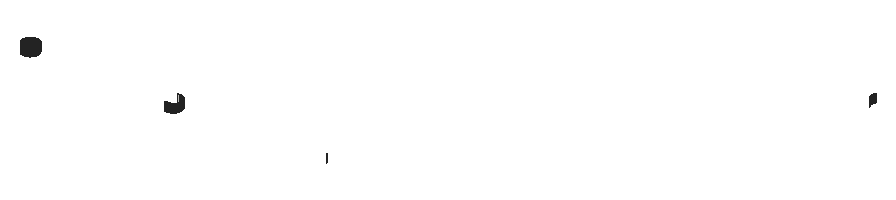
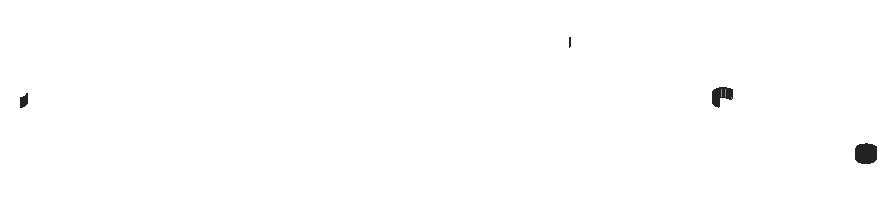
# SketchUp Ruby script. Lengths in inches.
U = 1.inch
M = Sketchup.active_model
def pt(a) = Geom::Point3d.new(a.map { |v| v * U })
def face(e, loops, mat)
  f = e.add_face(loops[0].map { |a| pt(a) })
  loops[1..].each { |l| e.add_face(l.map { |a| pt(a) }).erase! }
  f.material = f.back_material = mat if mat
  f
end
# faces: each face lists its corners as indices into pts; further lists are holes
def faces(e, pts, list, mat = nil) = list.each { |f| face(e, (f[0].is_a?(Array) ? f : [f]).map { |l| l.map { |i| pts[i] } }, mat) }
# xy, xz, yz: faces in a plane at the given z, y or x. An outline is a flat list of corners, or four numbers for a rectangle; further outlines are holes
def ring(l) = l.size == 4 ? [[l[0], l[1]], [l[2], l[1]], [l[2], l[3]], [l[0], l[3]]] : l.each_slice(2).to_a
def flat(e, list, mat, &to3) = list.each { |f| face(e, (f[0].is_a?(Array) ? f : [f]).map { |l| ring(l).map { |u, v| to3.(u, v) } }, mat) }
def xy(e, z, list, mat = nil) = flat(e, list, mat) { |x, y| [x, y, z] }
def xz(e, y, list, mat = nil) = flat(e, list, mat) { |x, z| [x, y, z] }
def yz(e, x, list, mat = nil) = flat(e, list, mat) { |y, z| [x, y, z] }
def lines(e, pts, list) = list.each { |a, b| e.add_line(pt(pts[a]), pt(pts[b])) }
# prism: a flat outline (further loops are holes) pulled along v
def prism(e, loops, v, mat = nil)
  f = face(e, loops, mat); d = Geom::Vector3d.new(v.map { |x| x * U })
  f.pushpull(f.normal.samedirection?(d) ? d.length : -d.length)
end
def box(e, o, s, mat = nil) = prism(e, [[o, [o[0] + s[0], o[1], o[2]], [o[0] + s[0], o[1] + s[1], o[2]], [o[0], o[1] + s[1], o[2]]]], [0, 0, s[2]], mat)
def at(x, y, z, deg = 0) = Geom::Transformation.translation(pt([x, y, z])) * Geom::Transformation.rotation(ORIGIN, Z_AXIS, deg.degrees)
def axes(o, x, y, z) = Geom::Transformation.new([*x, 0, *y, 0, *z, 0, *pt(o).to_a, 1])
def part(name) = M.definitions.add(name)
# library, detail: a bought-in or finely detailed component or shape, given as its bounding box
def library(name, o, s) = part(name).tap { |d| box(d.entities, o, s) }
def detail(e, o, s) = box(e.add_group.entities, o, s)
def put(e, d, t, mat = nil) = e.add_instance(d, t).tap { |i| i.material = mat if mat }
def group(e, t, mat = nil) = e.add_group.tap { |g| g.transformation = t; g.material = mat if mat }.entities
root = M.entities
xz(root,185,[[49.875,231,49.95,234],[49.95,231,50.03,234],[50.03,231,50.11,234],[104.68,231,104.75,234],[104.75,231,104.83,234],
  [104.83,231,104.91,234]])
xz(root,185.01,[[49.72,231,49.8,234],[50.19,231,50.27,234],[104.52,231,104.6,234],[104.99,231,105.07,234]])
xz(root,190.99,[[49.73,231,49.81,234],[50.2,231,50.28,234],[104.53,231,104.61,234],[105,231,105.08,234]])
xz(root,191,[[49.89,231,49.97,234],[49.97,231,50.05,234],[50.05,231,50.125,234],[104.6875,231,104.77,234],[104.77,231,104.85,234],
  [104.85,231,104.92,234]])
yz(root,47,[[187.89,231,187.97,234],[187.97,231,188.05,234],[188.05,231,188.125,234]])
yz(root,47.01,[[187.73,231,187.81,234],[188.2,231,188.28,234]])
yz(root,52.99,[[187.72,231,187.8,234],[188.19,231,188.27,234]])
yz(root,53,[[187.875,231,187.95,234],[187.95,231,188.03,234],[188.03,231,188.11,234]])
yz(root,107.79,[[187.72,231,187.8,234],[188.19,231,188.27,234]])
yz(root,107.8,[[187.875,231,187.95,234],[187.95,231,188.03,234],[188.03,231,188.11,234]])
yz(root,266.2,[[319.89,231,319.97,234],[319.97,231,320.05,234],[320.05,231,320.125,234]])
yz(root,266.21,[[319.73,231,319.81,234],[320.2,231,320.28,234]])
p = [[49.49,185.04,231],[49.41,185.06,231],[49.41,185.06,234],[49.49,185.04,234],[49.5625,185.03,231],[49.5625,185.03,234],
  [49.64,185.02,231],[49.64,185.02,234],[49.72,185.01,231],[49.72,185.01,234],[49.875,185,231],[49.8,185.01,231],
  [49.8,185.01,234],[49.875,185,234],[50.19,185.01,231],[50.11,185,231],[50.11,185,234],[50.19,185.01,234],
  [50.35,185.02,231],[50.27,185.01,231],[50.27,185.01,234],[50.35,185.02,234],[50.42,185.03,231],[50.42,185.03,234],
  [50.5,185.04,231],[50.5,185.04,234],[50.58,185.06,231],[50.58,185.06,234],[104.29,185.04,231],[104.21,185.06,231],
  [104.21,185.06,234],[104.29,185.04,234],[104.36,185.03,231],[104.36,185.03,234],[104.44,185.02,231],[104.44,185.02,234],
  [104.52,185.01,231],[104.52,185.01,234],[104.68,185,231],[104.6,185.01,231],[104.6,185.01,234],[104.68,185,234],
  [104.99,185.01,231],[104.91,185,231],[104.91,185,234],[104.99,185.01,234],[105.15,185.02,231],[105.07,185.01,231],
  [105.07,185.01,234],[105.15,185.02,234],[105.22,185.03,231],[105.22,185.03,234],[105.3,185.04,231],[105.3,185.04,234],
  [105.38,185.06,231],[105.38,185.06,234],[49.1,185.14,231],[49.03,185.16,231],[49.03,185.16,234],[49.1,185.14,234],
  [49.18,185.11,231],[49.18,185.11,234],[49.26,185.09,231],[49.26,185.09,234],[49.33,185.08,231],[49.33,185.08,234],
  [50.66,185.07,231],[50.66,185.07,234],[50.73,185.09,231],[50.73,185.09,234],[50.81,185.11,231],[50.81,185.11,234],
  [50.88,185.13,231],[50.88,185.13,234],[50.96,185.16,231],[50.96,185.16,234],[103.98,185.11,231],[103.9,185.14,231],
  [103.9,185.14,234],[103.98,185.11,234],[104.06,185.09,231],[104.06,185.09,234],[104.13,185.08,231],[104.13,185.08,234],
  [105.46,185.07,231],[105.46,185.07,234],[105.53,185.09,231],[105.53,185.09,234],[105.61,185.11,231],[105.61,185.11,234],
  [105.68,185.13,231],[105.68,185.13,234],[105.76,185.16,231],[105.76,185.16,234],[48.81,185.25,231],[48.74,185.28,231],
  [48.74,185.28,234],[48.81,185.25,234],[48.88,185.22,231],[48.88,185.22,234],[48.96,185.1875,231],[48.96,185.1875,234],
  [51.03,185.18,231],[51.03,185.18,234],[51.11,185.21,231],[51.11,185.21,234],[51.18,185.24,231],[51.18,185.24,234],
  [51.25,185.27,231],[51.25,185.27,234],[105.83,185.18,231],[105.83,185.18,234],[105.91,185.21,231],[105.91,185.21,234],
  [105.98,185.24,231],[105.98,185.24,234],[106.05,185.27,231],[106.05,185.27,234],[48.6,185.35,231],[48.53,185.39,231],
  [48.53,185.39,234],[48.6,185.35,234],[48.67,185.3125,231],[48.67,185.3125,234],[51.32,185.31,231],[51.32,185.31,234],
  [51.39,185.34,231],[51.39,185.34,234],[51.46,185.38,231],[51.46,185.38,234],[106.12,185.31,231],[106.12,185.31,234],
  [106.19,185.34,231],[106.19,185.34,234],[106.26,185.38,231],[106.26,185.38,234],[48.46,185.42,231],[48.39,185.47,231],
  [48.39,185.47,234],[48.46,185.42,234],[51.53,185.42,231],[51.53,185.42,234],[51.6,185.46,231],[51.6,185.46,234],
  [106.33,185.42,231],[106.33,185.42,234],[106.4,185.46,231],[106.4,185.46,234],[48.33,185.51,231],[48.26,185.55,231],
  [48.26,185.55,234],[48.33,185.51,234],[51.66,185.5,231],[51.66,185.5,234],[51.73,185.55,231],[51.73,185.55,234],
  [51.79,185.59,231],[51.79,185.59,234],[106.46,185.5,231],[106.46,185.5,234],[106.53,185.55,231],[106.53,185.55,234],
  [106.59,185.59,231],[106.59,185.59,234],[48.14,185.65,231],[48.08,185.7,231],[48.08,185.7,234],[48.14,185.65,234],
  [48.2,185.6,231],[48.2,185.6,234],[51.85,185.64,231],[51.85,185.64,234],[51.91,185.69,231],[51.91,185.69,234],
  [106.65,185.64,231],[106.65,185.64,234],[106.71,185.69,231],[106.71,185.69,234],[48.02,185.75,231],[47.96,185.8,231],
  [47.96,185.8,234],[48.02,185.75,234],[51.97,185.74,231],[51.97,185.74,234],[52.03,185.79,231],[52.03,185.79,234],
  [106.77,185.74,231],[106.77,185.74,234],[106.83,185.79,231],[106.83,185.79,234],[47.9,185.86,231],[47.9,185.86,234],
  [52.09,185.85,231],[52.09,185.85,234],[52.14,185.9,231],[52.14,185.9,234],[106.89,185.85,231],[106.89,185.85,234],
  [106.94,185.9,231],[106.94,185.9,234],[47.85,185.91,231],[47.79,185.97,231],[47.79,185.97,234],[47.85,185.91,234],
  [52.2,185.96,231],[52.2,185.96,234],[107,185.96,231],[107,185.96,234],[47.74,186.03,231],[47.69,186.09,231],
  [47.69,186.09,234],[47.74,186.03,234],[52.25,186.02,231],[52.25,186.02,234],[52.3,186.08,231],[52.3,186.08,234],
  [107.05,186.02,231],[107.05,186.02,234],[107.1,186.08,231],[107.1,186.08,234],[47.64,186.15,231],[47.59,186.21,231],
  [47.59,186.21,234],[47.64,186.15,234],[52.35,186.14,231],[52.35,186.14,234],[52.4,186.2,231],[52.4,186.2,234],
  [107.15,186.14,231],[107.15,186.14,234],[107.2,186.2,231],[107.2,186.2,234],[47.55,186.27,231],[47.55,186.27,234],
  [52.45,186.26,231],[52.45,186.26,234],[107.25,186.26,231],[107.25,186.26,234],[47.5,186.34,231],[47.46,186.4,231],
  [47.46,186.4,234],[47.5,186.34,234],[52.49,186.33,231],[52.49,186.33,234],[52.53,186.39,231],[52.53,186.39,234],
  [107.29,186.33,231],[107.29,186.33,234],[107.33,186.39,231],[107.33,186.39,234],[47.42,186.47,231],[47.42,186.47,234],
  [52.58,186.46,231],[52.58,186.46,234],[107.375,186.46,231],[107.375,186.46,234],[47.38,186.54,231],[47.34,186.61,231],
  [47.34,186.61,234],[47.38,186.54,234],[52.61,186.53,231],[52.61,186.53,234],[52.65,186.6,231],[52.65,186.6,234],
  [107.41,186.53,231],[107.41,186.53,234],[107.45,186.6,231],[107.45,186.6,234],[47.31,186.68,231],[47.31,186.68,234],
  [52.6875,186.67,231],[52.6875,186.67,234],[107.49,186.67,231],[107.49,186.67,234],[47.27,186.75,231],[47.24,186.82,231],
  [47.24,186.82,234],[47.27,186.75,234],[52.72,186.74,231],[52.72,186.74,234],[52.75,186.81,231],[52.75,186.81,234],
  [107.52,186.74,231],[107.52,186.74,234],[107.55,186.81,231],[107.55,186.81,234],[47.21,186.89,231],[47.21,186.89,234],
  [52.78,186.88,231],[52.78,186.88,234],[107.58,186.88,231],[107.58,186.88,234],[47.18,186.97,231],[47.18,186.97,234],
  [52.8125,186.96,231],[52.8125,186.96,234],[107.61,186.96,231],[107.61,186.96,234],[47.16,187.04,231],[47.13,187.12,231],
  [47.13,187.12,234],[47.16,187.04,234],[52.84,187.03,231],[52.84,187.03,234],[52.86,187.1,231],[52.86,187.1,234],
  [107.64,187.03,231],[107.64,187.03,234],[107.66,187.1,231],[107.66,187.1,234],[47.11,187.19,231],[47.11,187.19,234],
  [52.89,187.18,231],[52.89,187.18,234],[107.6875,187.18,231],[107.6875,187.18,234],[47.09,187.27,231],[47.09,187.27,234],
  [52.91,187.26,231],[52.91,187.26,234],[107.71,187.26,231],[107.71,187.26,234],[47.07,187.34,231],[47.06,187.42,231],
  [47.06,187.42,234],[47.07,187.34,234],[52.92,187.33,231],[52.92,187.33,234],[52.94,187.41,231],[52.94,187.41,234],
  [107.72,187.33,231],[107.72,187.33,234],[107.74,187.41,231],[107.74,187.41,234],[47.04,187.5,231],[47.04,187.5,234],
  [52.96,187.49,231],[52.96,187.49,234],[107.76,187.49,231],[107.76,187.49,234],[47.03,187.58,231],[47.03,187.58,234],
  [52.97,187.5625,231],[52.97,187.5625,234],[107.77,187.5625,231],[107.77,187.5625,234],[47.02,187.65,231],[47.02,187.65,234],
  [52.98,187.64,231],[52.98,187.64,234],[52.99,187.72,231],[52.99,187.72,234],[107.78,187.64,231],[107.78,187.64,234],
  [107.79,187.72,231],[107.79,187.72,234],[47.01,187.73,231],[47.01,187.73,234],[47.01,187.81,231],[47,187.89,231],
  [47,187.89,234],[47.01,187.81,234],[53,187.875,231],[52.99,187.8,231],[52.99,187.8,234],[53,187.875,234],
  [107.8,187.875,231],[107.79,187.8,231],[107.79,187.8,234],[107.8,187.875,234],[47,188.125,231],[47.01,188.2,231],
  [47.01,188.2,234],[47,188.125,234],[52.99,188.19,231],[53,188.11,231],[53,188.11,234],[52.99,188.19,234],
  [107.79,188.19,231],[107.8,188.11,231],[107.8,188.11,234],[107.79,188.19,234],[47.01,188.28,231],[47.02,188.36,231],
  [47.02,188.36,234],[47.01,188.28,234],[52.97,188.42,231],[52.98,188.35,231],[52.98,188.35,234],[52.97,188.42,234],
  [52.99,188.27,231],[52.99,188.27,234],[107.77,188.42,231],[107.78,188.35,231],[107.78,188.35,234],[107.77,188.42,234],
  [107.79,188.27,231],[107.79,188.27,234],[47.03,188.4375,231],[47.03,188.4375,234],[47.04,188.51,231],[47.04,188.51,234],
  [52.96,188.5,231],[52.96,188.5,234],[107.76,188.5,231],[107.76,188.5,234],[47.06,188.59,231],[47.06,188.59,234],
  [52.94,188.58,231],[52.94,188.58,234],[107.74,188.58,231],[107.74,188.58,234],[47.08,188.67,231],[47.08,188.67,234],
  [52.93,188.66,231],[52.93,188.66,234],[107.73,188.66,231],[107.73,188.66,234],[47.09,188.74,231],[47.09,188.74,234],
  [47.11,188.82,231],[47.11,188.82,234],[52.89,188.81,231],[52.91,188.73,231],[52.91,188.73,234],[52.89,188.81,234],
  [107.6875,188.81,231],[107.71,188.73,231],[107.71,188.73,234],[107.6875,188.81,234],[47.14,188.9,231],[47.14,188.9,234],
  [52.87,188.88,231],[52.87,188.88,234],[107.67,188.88,231],[107.67,188.88,234],[47.16,188.97,231],[47.16,188.97,234],
  [52.84,188.96,231],[52.84,188.96,234],[107.64,188.96,231],[107.64,188.96,234],[47.1875,189.04,231],[47.1875,189.04,234],
  [47.22,189.12,231],[47.22,189.12,234],[52.79,189.11,231],[52.82,189.03,231],[52.82,189.03,234],[52.79,189.11,234],
  [107.59,189.11,231],[107.62,189.03,231],[107.62,189.03,234],[107.59,189.11,234],[47.25,189.19,231],[47.25,189.19,234],
  [52.76,189.18,231],[52.76,189.18,234],[107.56,189.18,231],[107.56,189.18,234],[47.28,189.26,231],[47.28,189.26,234],
  [52.73,189.25,231],[52.73,189.25,234],[107.53,189.25,231],[107.53,189.25,234],[47.3125,189.33,231],[47.3125,189.33,234],
  [47.35,189.4,231],[47.35,189.4,234],[52.66,189.39,231],[52.69,189.32,231],[52.69,189.32,234],[52.66,189.39,234],
  [107.46,189.39,231],[107.49,189.32,231],[107.49,189.32,234],[107.46,189.39,234],[47.39,189.47,231],[47.39,189.47,234],
  [52.62,189.46,231],[52.62,189.46,234],[107.42,189.46,231],[107.42,189.46,234],[47.42,189.54,231],[47.42,189.54,234],
  [47.47,189.61,231],[47.47,189.61,234],[52.54,189.6,231],[52.58,189.53,231],[52.58,189.53,234],[52.54,189.6,234],
  [107.34,189.6,231],[107.38,189.53,231],[107.38,189.53,234],[107.34,189.6,234],[47.51,189.67,231],[47.51,189.67,234],
  [52.5,189.66,231],[52.5,189.66,234],[107.3,189.66,231],[107.3,189.66,234],[47.55,189.74,231],[47.55,189.74,234],
  [47.6,189.8,231],[47.6,189.8,234],[52.41,189.79,231],[52.45,189.73,231],[52.45,189.73,234],[52.41,189.79,234],
  [107.21,189.79,231],[107.25,189.73,231],[107.25,189.73,234],[107.21,189.79,234],[47.65,189.86,231],[47.65,189.86,234],
  [52.36,189.85,231],[52.36,189.85,234],[107.16,189.85,231],[107.16,189.85,234],[47.7,189.92,231],[47.7,189.92,234],
  [47.75,189.98,231],[47.75,189.98,234],[52.26,189.97,231],[52.31,189.91,231],[52.31,189.91,234],[52.26,189.97,234],
  [107.06,189.97,231],[107.11,189.91,231],[107.11,189.91,234],[107.06,189.97,234],[47.8,190.04,231],[47.8,190.04,234],
  [47.86,190.1,231],[47.86,190.1,234],[52.15,190.09,231],[52.21,190.03,231],[52.21,190.03,234],[52.15,190.09,234],
  [106.95,190.09,231],[107.01,190.03,231],[107.01,190.03,234],[106.95,190.09,234],[47.91,190.15,231],[47.91,190.15,234],
  [52.04,190.2,231],[52.1,190.14,231],[52.1,190.14,234],[52.04,190.2,234],[106.84,190.2,231],[106.9,190.14,231],
  [106.9,190.14,234],[106.84,190.2,234],[47.97,190.21,231],[47.97,190.21,234],[48.03,190.26,231],[48.03,190.26,234],
  [51.98,190.25,231],[51.98,190.25,234],[106.78,190.25,231],[106.78,190.25,234],[48.09,190.31,231],[48.09,190.31,234],
  [48.15,190.36,231],[48.15,190.36,234],[51.86,190.35,231],[51.92,190.3,231],[51.92,190.3,234],[51.86,190.35,234],
  [106.66,190.35,231],[106.72,190.3,231],[106.72,190.3,234],[106.66,190.35,234],[161.46,190.35,231],[161.52,190.3,231],
  [161.52,190.3,234],[161.46,190.35,234],[161.58,190.25,231],[161.58,190.25,234],[48.21,190.41,231],[48.21,190.41,234],
  [48.27,190.45,231],[48.27,190.45,234],[51.67,190.49,231],[51.74,190.45,231],[51.74,190.45,234],[51.67,190.49,234],
  [51.8,190.4,231],[51.8,190.4,234],[106.47,190.49,231],[106.54,190.45,231],[106.54,190.45,234],[106.47,190.49,234],
  [106.6,190.4,231],[106.6,190.4,234],[161.4,190.4,231],[161.4,190.4,234],[48.34,190.5,231],[48.34,190.5,234],
  [48.4,190.54,231],[48.4,190.54,234],[48.47,190.58,231],[48.47,190.58,234],[51.54,190.58,231],[51.61,190.53,231],
  [51.61,190.53,234],[51.54,190.58,234],[106.34,190.58,231],[106.41,190.53,231],[106.41,190.53,234],[106.34,190.58,234],
  [48.54,190.62,231],[48.54,190.62,234],[48.61,190.66,231],[48.61,190.66,234],[51.4,190.65,231],[51.47,190.61,231],
  [51.47,190.61,234],[51.4,190.65,234],[106.2,190.65,231],[106.27,190.61,231],[106.27,190.61,234],[106.2,190.65,234],
  [48.68,190.69,231],[48.68,190.69,234],[48.75,190.73,231],[48.75,190.73,234],[48.82,190.76,231],[48.82,190.76,234],
  [51.19,190.75,231],[51.26,190.72,231],[51.26,190.72,234],[51.19,190.75,234],[51.33,190.6875,231],[51.33,190.6875,234],
  [105.99,190.75,231],[106.0625,190.72,231],[106.0625,190.72,234],[105.99,190.75,234],[106.13,190.6875,231],[106.13,190.6875,234],
  [48.89,190.79,231],[48.89,190.79,234],[48.97,190.82,231],[48.97,190.82,234],[49.04,190.84,231],[49.04,190.84,234],
  [49.12,190.87,231],[49.12,190.87,234],[50.9,190.86,231],[50.97,190.84,231],[50.97,190.84,234],[50.9,190.86,234],
  [51.04,190.8125,231],[51.04,190.8125,234],[51.12,190.78,231],[51.12,190.78,234],[105.7,190.86,231],[105.77,190.84,231],
  [105.77,190.84,234],[105.7,190.86,234],[105.84,190.8125,231],[105.84,190.8125,234],[105.92,190.78,231],[105.92,190.78,234],
  [49.19,190.89,231],[49.19,190.89,234],[49.27,190.91,231],[49.27,190.91,234],[49.34,190.93,231],[49.34,190.93,234],
  [49.42,190.94,231],[49.42,190.94,234],[49.5,190.96,231],[49.5,190.96,234],[50.51,190.96,231],[50.59,190.94,231],
  [50.59,190.94,234],[50.51,190.96,234],[50.67,190.92,231],[50.67,190.92,234],[50.74,190.91,231],[50.74,190.91,234],
  [50.82,190.89,231],[50.82,190.89,234],[103.92,190.87,231],[103.99,190.89,231],[103.99,190.89,234],[103.92,190.87,234],
  [104.07,190.91,231],[104.07,190.91,234],[104.14,190.93,231],[104.14,190.93,234],[104.22,190.94,231],[104.22,190.94,234],
  [104.3,190.96,231],[104.3,190.96,234],[105.3125,190.96,231],[105.39,190.94,231],[105.39,190.94,234],[105.3125,190.96,234],
  [105.47,190.92,231],[105.47,190.92,234],[105.54,190.91,231],[105.54,190.91,234],[105.62,190.89,231],[105.62,190.89,234],
  [49.58,190.97,231],[49.58,190.97,234],[49.65,190.98,231],[49.65,190.98,234],[49.73,190.99,231],[49.73,190.99,234],
  [49.81,190.99,231],[49.89,191,231],[49.89,191,234],[49.81,190.99,234],[50.125,191,231],[50.2,190.99,231],
  [50.2,190.99,234],[50.125,191,234],[50.28,190.99,231],[50.36,190.98,231],[50.36,190.98,234],[50.28,190.99,234],
  [50.4375,190.97,231],[50.4375,190.97,234],[104.375,190.97,231],[104.375,190.97,234],[104.45,190.98,231],[104.45,190.98,234],
  [104.53,190.99,231],[104.53,190.99,234],[104.61,190.99,231],[104.6875,191,231],[104.6875,191,234],[104.61,190.99,234],
  [104.92,191,231],[105,190.99,231],[105,190.99,234],[104.92,191,234],[105.08,190.99,231],[105.16,190.98,231],
  [105.16,190.98,234],[105.08,190.99,234],[105.24,190.97,231],[105.24,190.97,234],[266.66,318.4,231],[266.62,318.47,231],
  [266.62,318.47,234],[266.66,318.4,234],[266.58,318.54,231],[266.54,318.61,231],[266.54,318.61,234],[266.58,318.54,234],
  [266.51,318.68,231],[266.51,318.68,234],[266.47,318.75,231],[266.44,318.82,231],[266.44,318.82,234],[266.47,318.75,234],
  [266.41,318.89,231],[266.41,318.89,234],[266.38,318.97,231],[266.38,318.97,234],[266.36,319.04,231],[266.33,319.12,231],
  [266.33,319.12,234],[266.36,319.04,234],[266.3125,319.19,231],[266.3125,319.19,234],[266.29,319.27,231],[266.29,319.27,234],
  [266.27,319.34,231],[266.26,319.42,231],[266.26,319.42,234],[266.27,319.34,234],[266.24,319.5,231],[266.24,319.5,234],
  [266.23,319.58,231],[266.23,319.58,234],[266.22,319.65,231],[266.22,319.65,234],[266.21,319.73,231],[266.21,319.73,234],
  [266.21,319.81,231],[266.2,319.89,231],[266.2,319.89,234],[266.21,319.81,234],[266.2,320.125,231],[266.21,320.2,231],
  [266.21,320.2,234],[266.2,320.125,234],[266.21,320.28,231],[266.22,320.36,231],[266.22,320.36,234],[266.21,320.28,234],
  [266.23,320.4375,231],[266.23,320.4375,234],[266.24,320.51,231],[266.24,320.51,234],[266.26,320.59,231],[266.26,320.59,234],
  [266.28,320.67,231],[266.28,320.67,234],[266.29,320.74,231],[266.29,320.74,234],[266.3125,320.82,231],[266.3125,320.82,234],
  [266.34,320.9,231],[266.34,320.9,234],[266.36,320.97,231],[266.36,320.97,234],[266.39,321.04,231],[266.39,321.04,234],
  [266.42,321.12,231],[266.42,321.12,234],[266.45,321.19,231],[266.45,321.19,234],[266.48,321.26,231],[266.48,321.26,234],
  [266.51,321.33,231],[266.51,321.33,234],[266.55,321.4,231],[266.55,321.4,234],[266.59,321.47,231],[266.59,321.47,234],
  [266.625,321.54,231],[266.625,321.54,234],[266.67,321.61,231],[266.67,321.61,234]]
faces(root,p,[[0,1,2,3],[4,0,3,5],[6,4,5,7],[8,6,7,9],[10,11,12,13],[14,15,16,17],[18,19,20,21],[22,18,21,23],
  [24,22,23,25],[26,24,25,27],[28,29,30,31],[32,28,31,33],[34,32,33,35],[36,34,35,37],[38,39,40,41],[42,43,44,45],
  [46,47,48,49],[50,46,49,51],[52,50,51,53],[54,52,53,55],[56,57,58,59],[60,56,59,61],[62,60,61,63],[64,62,63,65],
  [1,64,65,2],[66,26,27,67],[68,66,67,69],[70,68,69,71],[72,70,71,73],[74,72,73,75],[76,77,78,79],[80,76,79,81],
  [82,80,81,83],[29,82,83,30],[84,54,55,85],[86,84,85,87],[88,86,87,89],[90,88,89,91],[92,90,91,93],[94,95,96,97],
  [98,94,97,99],[100,98,99,101],[57,100,101,58],[102,74,75,103],[104,102,103,105],[106,104,105,107],[108,106,107,109],[110,92,93,111],
  [112,110,111,113],[114,112,113,115],[116,114,115,117],[118,119,120,121],[122,118,121,123],[95,122,123,96],[124,108,109,125],[126,124,125,127],
  [128,126,127,129],[130,116,117,131],[132,130,131,133],[134,132,133,135],[136,137,138,139],[119,136,139,120],[140,128,129,141],[142,140,141,143],
  [144,134,135,145],[146,144,145,147],[148,149,150,151],[137,148,151,138],[152,142,143,153],[154,152,153,155],[156,154,155,157],[158,146,147,159],
  [160,158,159,161],[162,160,161,163],[164,165,166,167],[168,164,167,169],[149,168,169,150],[170,156,157,171],[172,170,171,173],[174,162,163,175],
  [176,174,175,177],[178,179,180,181],[165,178,181,166],[182,172,173,183],[184,182,183,185],[186,176,177,187],[188,186,187,189],[179,190,191,180],
  [192,184,185,193],[194,192,193,195],[196,188,189,197],[198,196,197,199],[200,201,202,203],[190,200,203,191],[204,194,195,205],[206,198,199,207],
  [208,209,210,211],[201,208,211,202],[212,204,205,213],[214,212,213,215],[216,206,207,217],[218,216,217,219],[220,221,222,223],[209,220,223,210],
  [224,214,215,225],[226,224,225,227],[228,218,219,229],[230,228,229,231],[221,232,233,222],[234,226,227,235],[236,230,231,237],[238,239,240,241],
  [232,238,241,233],[242,234,235,243],[244,242,243,245],[246,236,237,247],[248,246,247,249],[239,250,251,240],[252,244,245,253],[254,248,249,255],
  [256,257,258,259],[250,256,259,251],[260,252,253,261],[262,260,261,263],[264,254,255,265],[266,264,265,267],[257,268,269,258],[270,262,263,271],
  [272,266,267,273],[274,275,276,277],[268,274,277,269],[278,270,271,279],[280,278,279,281],[282,272,273,283],[284,282,283,285],[275,286,287,276],
  [288,280,281,289],[290,284,285,291],[286,292,293,287],[294,288,289,295],[296,290,291,297],[298,299,300,301],[292,298,301,293],[302,294,295,303],
  [304,302,303,305],[306,296,297,307],[308,306,307,309],[299,310,311,300],[312,304,305,313],[314,308,309,315],[310,316,317,311],[318,312,313,319],
  [320,314,315,321],[322,323,324,325],[316,322,325,317],[326,318,319,327],[328,326,327,329],[330,320,321,331],[332,330,331,333],[323,334,335,324],
  [336,328,329,337],[338,332,333,339],[334,340,341,335],[342,336,337,343],[344,338,339,345],[340,346,347,341],[348,342,343,349],[350,348,349,351],
  [352,344,345,353],[354,352,353,355],[346,356,357,347],[358,359,360,361],[362,363,364,365],[366,367,368,369],[370,371,372,373],[374,375,376,377],
  [378,379,380,381],[382,383,384,385],[386,387,388,389],[387,390,391,388],[392,393,394,395],[393,396,397,394],[383,398,399,384],[398,400,401,399],
  [402,386,389,403],[404,392,395,405],[400,406,407,401],[408,402,403,409],[410,404,405,411],[406,412,413,407],[414,408,409,415],[416,410,411,417],
  [412,418,419,413],[418,420,421,419],[422,423,424,425],[423,414,415,424],[426,427,428,429],[427,416,417,428],[420,430,431,421],[432,422,425,433],
  [434,426,429,435],[430,436,437,431],[438,432,433,439],[440,434,435,441],[436,442,443,437],[442,444,445,443],[446,447,448,449],[447,438,439,448],
  [450,451,452,453],[451,440,441,452],[444,454,455,445],[456,446,449,457],[458,450,453,459],[454,460,461,455],[462,456,457,463],[464,458,459,465],
  [460,466,467,461],[466,468,469,467],[470,471,472,473],[471,462,463,472],[474,475,476,477],[475,464,465,476],[468,478,479,469],[480,470,473,481],
  [482,474,477,483],[478,484,485,479],[484,486,487,485],[488,489,490,491],[489,480,481,490],[492,493,494,495],[493,482,483,494],[486,496,497,487],
  [498,488,491,499],[500,492,495,501],[496,502,503,497],[502,504,505,503],[506,507,508,509],[507,498,499,508],[510,511,512,513],[511,500,501,512],
  [504,514,515,505],[516,506,509,517],[518,510,513,519],[514,520,521,515],[520,522,523,521],[524,525,526,527],[525,516,517,526],[528,529,530,531],
  [529,518,519,530],[522,532,533,523],[532,534,535,533],[536,537,538,539],[537,524,527,538],[540,541,542,543],[541,528,531,542],[534,544,545,535],
  [546,547,548,549],[547,536,539,548],[550,551,552,553],[551,540,543,552],[544,554,555,545],[554,556,557,555],[558,546,549,559],[560,550,553,561],
  [556,562,563,557],[562,564,565,563],[566,567,568,569],[567,558,559,568],[570,571,572,573],[571,560,561,572],[574,575,576,577],[575,578,579,576],
  [564,580,581,565],[580,582,583,581],[584,585,586,587],[585,588,589,586],[588,566,569,589],[590,591,592,593],[591,594,595,592],[594,570,573,595],
  [596,574,577,597],[582,598,599,583],[598,600,601,599],[600,602,603,601],[604,605,606,607],[605,584,587,606],[608,609,610,611],[609,590,593,610],
  [602,612,613,603],[612,614,615,613],[616,617,618,619],[617,604,607,618],[620,621,622,623],[621,608,611,622],[614,624,625,615],[624,626,627,625],
  [626,628,629,627],[630,631,632,633],[631,634,635,632],[634,616,619,635],[636,637,638,639],[637,640,641,638],[640,620,623,641],[628,642,643,629],
  [642,644,645,643],[644,646,647,645],[646,648,649,647],[650,651,652,653],[651,654,655,652],[654,656,657,655],[656,630,633,657],[658,659,660,661],
  [659,662,663,660],[662,664,665,663],[664,636,639,665],[648,666,667,649],[666,668,669,667],[668,670,671,669],[670,672,673,671],[672,674,675,673],
  [676,677,678,679],[677,680,681,678],[680,682,683,681],[682,684,685,683],[684,650,653,685],[686,687,688,689],[687,690,691,688],[690,692,693,691],
  [692,694,695,693],[694,696,697,695],[698,699,700,701],[699,702,703,700],[702,704,705,703],[704,706,707,705],[706,658,661,707],[674,708,709,675],
  [708,710,711,709],[710,712,713,711],[714,715,716,717],[718,719,720,721],[722,723,724,725],[723,726,727,724],[726,676,679,727],[696,728,729,697],
  [728,730,731,729],[730,732,733,731],[734,735,736,737],[738,739,740,741],[742,743,744,745],[743,746,747,744],[746,698,701,747],[748,749,750,751],
  [752,753,754,755],[749,752,755,750],[753,756,757,754],[758,759,760,761],[756,758,761,757],[759,762,763,760],[762,764,765,763],[766,767,768,769],
  [764,766,769,765],[767,770,771,768],[770,772,773,771],[774,775,776,777],[772,774,777,773],[775,778,779,776],[778,780,781,779],[780,782,783,781],
  [782,784,785,783],[786,787,788,789],[790,791,792,793],[794,795,796,797],[795,798,799,796],[798,800,801,799],[800,802,803,801],[802,804,805,803],
  [804,806,807,805],[806,808,809,807],[808,810,811,809],[810,812,813,811],[812,814,815,813],[814,816,817,815],[816,818,819,817],[818,820,821,819],
  [820,822,823,821],[822,824,825,823],[824,826,827,825],[826,828,829,827],[828,830,831,829]])
